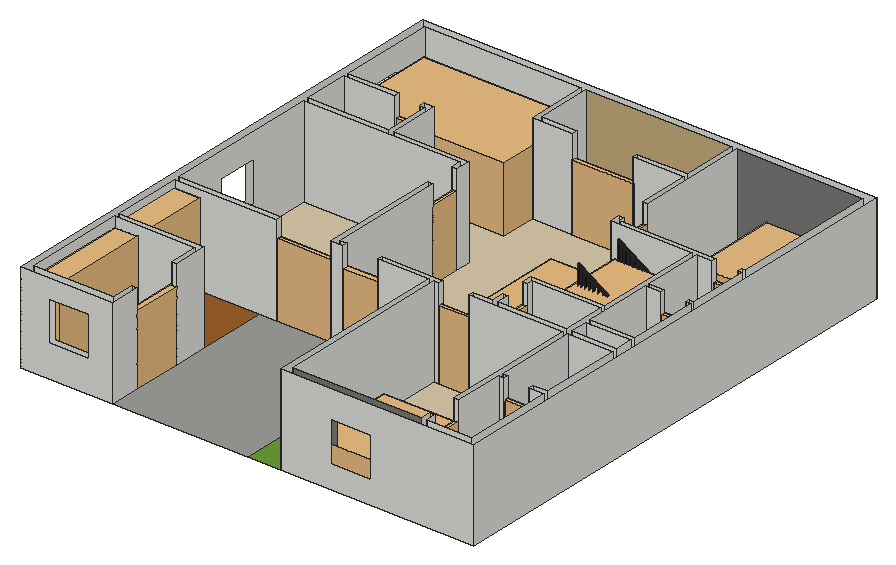
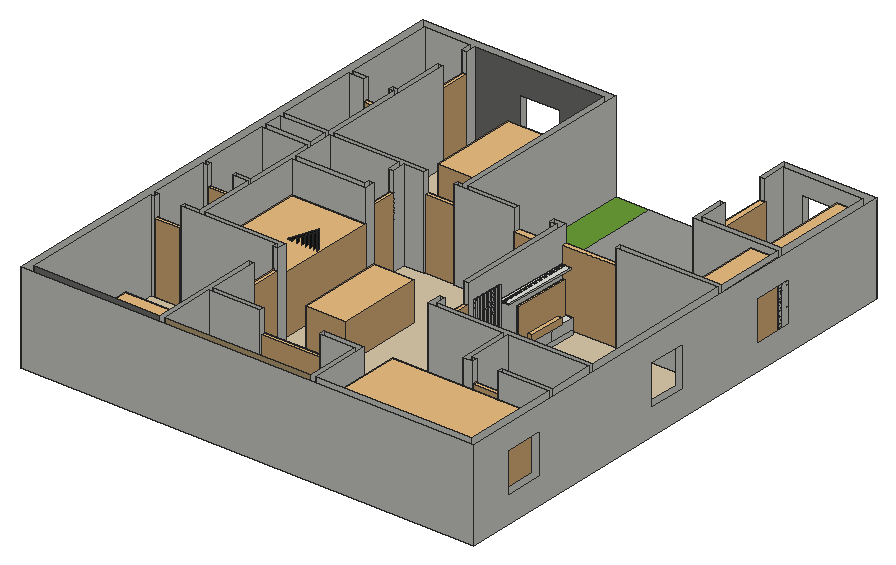
# SketchUp Ruby script. Lengths in inches.
U = 1.inch
M = Sketchup.active_model
def pt(a) = Geom::Point3d.new(a.map { |v| v * U })
def face(e, loops, mat)
  f = e.add_face(loops[0].map { |a| pt(a) })
  loops[1..].each { |l| e.add_face(l.map { |a| pt(a) }).erase! }
  f.material = f.back_material = mat if mat
  f
end
# faces: each face lists its corners as indices into pts; further lists are holes
def faces(e, pts, list, mat = nil) = list.each { |f| face(e, (f[0].is_a?(Array) ? f : [f]).map { |l| l.map { |i| pts[i] } }, mat) }
# xy, xz, yz: faces in a plane at the given z, y or x. An outline is a flat list of corners, or four numbers for a rectangle; further outlines are holes
def ring(l) = l.size == 4 ? [[l[0], l[1]], [l[2], l[1]], [l[2], l[3]], [l[0], l[3]]] : l.each_slice(2).to_a
def flat(e, list, mat, &to3) = list.each { |f| face(e, (f[0].is_a?(Array) ? f : [f]).map { |l| ring(l).map { |u, v| to3.(u, v) } }, mat) }
def xy(e, z, list, mat = nil) = flat(e, list, mat) { |x, y| [x, y, z] }
def xz(e, y, list, mat = nil) = flat(e, list, mat) { |x, z| [x, y, z] }
def yz(e, x, list, mat = nil) = flat(e, list, mat) { |y, z| [x, y, z] }
def lines(e, pts, list) = list.each { |a, b| e.add_line(pt(pts[a]), pt(pts[b])) }
# prism: a flat outline (further loops are holes) pulled along v
def prism(e, loops, v, mat = nil)
  f = face(e, loops, mat); d = Geom::Vector3d.new(v.map { |x| x * U })
  f.pushpull(f.normal.samedirection?(d) ? d.length : -d.length)
end
def box(e, o, s, mat = nil) = prism(e, [[o, [o[0] + s[0], o[1], o[2]], [o[0] + s[0], o[1] + s[1], o[2]], [o[0], o[1] + s[1], o[2]]]], [0, 0, s[2]], mat)
def at(x, y, z, deg = 0) = Geom::Transformation.translation(pt([x, y, z])) * Geom::Transformation.rotation(ORIGIN, Z_AXIS, deg.degrees)
def axes(o, x, y, z) = Geom::Transformation.new([*x, 0, *y, 0, *z, 0, *pt(o).to_a, 1])
def part(name) = M.definitions.add(name)
# library, detail: a bought-in or finely detailed component or shape, given as its bounding box
def library(name, o, s) = part(name).tap { |d| box(d.entities, o, s) }
def detail(e, o, s) = box(e.add_group.entities, o, s)
def put(e, d, t, mat = nil) = e.add_instance(d, t).tap { |i| i.material = mat if mat }
def group(e, t, mat = nil) = e.add_group.tap { |g| g.transformation = t; g.material = mat if mat }.entities
root = M.entities
M.materials.add("[Concrete Block 8x8 Gray]").color = [157, 158, 154]
M.materials.add("[Encaustic Tile Circular 01]").color = [123, 123, 122]
M.materials.add("[Field Square Tile]").color = [217, 201, 169]
M.materials.add("[Grass Dark Green]").color = [106, 157, 55]
M.materials.add("[Metal Panel]").color = [143, 157, 158]
M.materials.add("[Metal_Aluminum_Anodized]").color = [200, 209, 218]
M.materials.add("[Metal_Seamed]").color = [25, 25, 24]
M.materials.add("[Roofing Slate Tan]").color = [200, 175, 128]
M.materials.add("[Wood Floor Dark]").color = [153, 94, 42]
c1 = library("door",[0,0,0],[36,4.39,84])
c2 = library("double Door",[0,0,0],[79.98,10,87.99])
c3 = library("Gruppe\#1",[0,8.87,0],[102.36,152.23,141.73])
c4 = part("stairs, Holztreppe")
p = [[-31.58,140.69,125.98],[-31.58,140.71,125.98]]
lines(c4.entities,p,[[0,1]])
put(c4.entities,c3,axes([-51.18,-74.49,0],[1,0,0],[0,1,0],[0,0,0.77775]))
c5 = part("Group\#71")
box(c5.entities,[0,0,0],[1.97,1.22,32.37],"[Metal_Seamed]")
c6 = part("Group\#81")
box(c6.entities,[0,0,0],[1.97,51.19,3.0625],"[Metal_Seamed]")
c7 = part("Group\#76")
prism(c7.entities,[[[1.97,94.48,0],[1.97,94.48,3.0625],[1.97,0,58.18],[1.97,0,55.12]]],[-1.97,0,0],"[Metal_Seamed]")
c8 = part("Group\#74")
xz(c8.entities,0,[[0,0,1.97,33.27]],"[Metal_Seamed]")
xz(c8.entities,1.02,[[0,0,1.97,32.68]],"[Metal_Seamed]")
yz(c8.entities,0,[[0,0,0,33.27,1.02,32.68,1.02,0]],"[Metal_Seamed]")
yz(c8.entities,1.97,[[0,0,1.02,0,1.02,32.68,0,33.27]],"[Metal_Seamed]")
c9 = part("Group\#86")
box(c9.entities,[0,0,0],[1.18,1.97,32.37],"[Metal_Seamed]")
c10 = part("Untitled")
g1 = group(c10.entities,at(-2.72,-61.9,-3.0625))
g2 = group(g1,at(0,0,0))
put(g2,c4,at(53.15,65.62,3.0625))
g3 = group(g2,at(0,6.55,0))
g4 = group(g3,at(0,94.49,55.12))
xy(g4,0,[[104.33,0,106.3,51.19],[0,51.19,106.3,53.16]],"[Metal_Seamed]")
xy(g4,3.0625,[[104.33,0,106.3,8.07],[104.33,9.29,106.3,51.19],[0,51.19,106.3,53.16]],"[Metal_Seamed]")
xz(g4,0,[[104.33,0,106.3,3.0625]],"[Metal_Seamed]")
xz(g4,51.19,[[0,0,104.33,3.0625],[104.33,0,106.3,3.0625]],"[Metal_Seamed]")
xz(g4,53.16,[[0,0,106.3,3.0625]],"[Metal_Seamed]")
yz(g4,0,[[51.19,0,53.16,3.0625]],"[Metal_Seamed]")
yz(g4,104.33,[[0,0,51.19,3.0625]],"[Metal_Seamed]")
yz(g4,106.3,[[0,0,51.19,3.0625],[51.19,0,53.16,3.0625]],"[Metal_Seamed]")
put(g4,c5,at(104.33,8.07,3.0625))
put(g4,c5,at(104.33,19.6,3.0625))
put(g4,c5,at(104.33,30.24,3.0625))
put(g4,c5,at(104.33,40.72,3.0625))
put(g4,c5,at(104.33,51.95,3.0625))
put(g4,c5,at(0,51.89,3.0625))
put(g4,c5,at(0,8.01,3.0625))
put(g4,c5,at(0,19.54,3.0625))
put(g4,c5,at(0,40.66,3.0625))
put(g4,c5,at(0,30.18,3.0625))
put(g3,c6,at(0,94.49,55.12))
put(g3,c7,at(0,0.01,55.12))
g5 = group(g3,at(104.33,0.01,58.18))
prism(g5,[[[1.97,0,-55.12],[1.97,1.02,-54.52],[1.97,94.48,0],[1.97,94.48,-3.0625],[1.97,0,-58.18]]],[-1.97,0,0],"[Metal_Seamed]")
xy(g5,-21.84,[[0,0,1.97,1.02]],"[Metal_Seamed]")
put(g5,c8,axes([0,0,-21.84],[1,0,0],[0,1,0],[0,0,-1]))
put(g5,c8,axes([0,7.26,-17.61],[1,0,0],[0,1,0],[0,0,-1]))
put(g5,c8,axes([0,14.83,-13.19],[1,0,0],[0,1,0],[0,0,-1]))
put(g5,c8,axes([0,23.44,-8.17],[1,0,0],[0,1,0],[0,0,-1]))
put(g5,c8,axes([0,32.28,-3.01],[1,0,0],[0,1,0],[0,0,-1]))
put(g5,c8,axes([0,41.76,2.52],[1,0,0],[0,1,0],[0,0,-1]))
put(g5,c8,axes([0,51.4,8.14],[1,0,0],[0,1,0],[0,0,-1]))
put(g5,c8,axes([0,61.47,14.02],[1,0,0],[0,1,0],[0,0,-1]))
put(g5,c8,axes([0,72,20.16],[1,0,0],[0,1,0],[0,0,-1]))
put(g5,c8,axes([0,81.86,25.91],[1,0,0],[0,1,0],[0,0,-1]))
put(g5,c8,axes([0,93.45,32.68],[1,0,0],[0,1,0],[0,0,-1]))
put(g5,c8,axes([-49.33,51.4,8.14],[1,0,0],[0,1,0],[0,0,-1]))
put(g5,c8,axes([-49.33,93.45,32.68],[1,0,0],[0,1,0],[0,0,-1]))
put(g5,c8,axes([-49.33,0,-21.84],[1,0,0],[0,1,0],[0,0,-1]))
put(g5,c8,axes([-49.33,41.76,2.52],[1,0,0],[0,1,0],[0,0,-1]))
put(g5,c8,axes([-49.33,72,20.16],[1,0,0],[0,1,0],[0,0,-1]))
put(g5,c8,axes([-49.33,32.28,-3.01],[1,0,0],[0,1,0],[0,0,-1]))
put(g5,c8,axes([-49.33,23.44,-8.17],[1,0,0],[0,1,0],[0,0,-1]))
put(g5,c8,axes([-49.33,81.86,25.91],[1,0,0],[0,1,0],[0,0,-1]))
put(g5,c8,axes([-49.33,14.83,-13.19],[1,0,0],[0,1,0],[0,0,-1]))
put(g5,c8,axes([-49.33,61.47,14.02],[1,0,0],[0,1,0],[0,0,-1]))
put(g5,c8,axes([-49.33,7.26,-17.61],[1,0,0],[0,1,0],[0,0,-1]))
put(g5,c8,at(-104.33,93.45,-0.18))
put(g5,c8,at(-104.33,23.44,40.66))
put(g5,c8,at(-104.33,7.26,50.11))
put(g5,c8,at(-104.33,72,12.34))
put(g5,c8,at(-104.33,32.28,35.51))
put(g5,c8,at(-104.33,0,54.34))
put(g5,c8,at(-104.33,81.86,6.59))
put(g5,c8,at(-104.33,14.83,45.6875))
put(g5,c8,at(-104.33,61.47,18.48))
put(g5,c8,at(-104.33,41.76,29.97))
put(g5,c8,at(-104.33,51.4,24.35))
put(g5,c8,at(-55.12,23.43,40.26))
put(g5,c8,at(-55.12,81.84,6.18))
put(g5,c8,at(-55.12,7.24,49.7))
put(g5,c8,at(-55.12,-0.01,53.93))
put(g5,c8,at(-55.12,41.75,29.57))
put(g5,c8,at(-55.12,61.46,18.07))
put(g5,c8,at(-55.12,93.44,-0.59))
put(g5,c8,at(-55.12,32.27,35.1))
put(g5,c8,at(-55.12,51.39,23.95))
put(g5,c8,at(-55.12,14.8125,45.29))
put(g5,c8,at(-55.12,71.98,11.93))
put(g3,c7,at(49.21,0,55.12))
put(g3,c7,axes([55,0.01,58.18],[1,0,0],[0,1,0],[0,0,-1]))
g6 = group(g2,at(0,6.55,35.43))
p = [[51.18,94.48,55.12],[51.18,94.48,58.18],[55,94.49,58.18],[55,94.49,55.12]]
faces(g6,p,[[0,1,2,3]],"[Metal_Seamed]")
g7 = group(g6,at(0,94.49,55.12))
xy(g7,0,[[104.33,0,106.3,51.19],[0,51.19,106.3,53.16]],"[Metal_Seamed]")
xy(g7,3.0625,[[104.33,0,106.3,51.19],[0,51.19,106.3,53.16]],"[Metal_Seamed]")
xz(g7,0,[[104.33,0,106.3,3.0625]],"[Metal_Seamed]")
xz(g7,51.19,[[0,0,104.33,3.0625],[104.33,0,106.3,3.0625]],"[Metal_Seamed]")
xz(g7,53.16,[[0,0,106.3,3.0625]],"[Metal_Seamed]")
yz(g7,0,[[51.19,0,53.16,3.0625]],"[Metal_Seamed]")
yz(g7,104.33,[[0,0,51.19,3.0625]],"[Metal_Seamed]")
yz(g7,106.3,[[0,0,51.19,3.0625],[51.19,0,53.16,3.0625]],"[Metal_Seamed]")
put(g6,c6,at(0,94.49,55.12))
put(g6,c7,at(0,0.01,55.12))
put(g6,c7,axes([104.33,0.01,58.18],[1,0,0],[0,1,0],[0,0,-1]))
put(g6,c7,at(49.21,0,55.12))
put(g6,c7,axes([55,0.01,58.18],[1,0,0],[0,1,0],[0,0,-1]))
put(g1,c9,at(94.51,152.23,58.18))
put(g1,c9,at(48.39,152.23,58.18))
put(g1,c9,at(21.29,152.23,58.18))
put(g1,c9,at(85.01,152.23,58.18))
put(g1,c9,at(58.09,152.23,58.18))
put(g1,c9,at(75.58,152.23,58.18))
put(g1,c9,at(66.57,152.23,58.18))
put(g1,c9,at(38.93,152.23,58.18))
put(g1,c9,at(10.71,152.23,58.18))
put(g1,c9,at(29.75,152.23,58.18))
c11 = library("sliding+window",[0,-1.1,0],[78.74,4.33,80.71])
c12 = library("door1",[3.7,-4.82,1.36],[53.55,7.65,83.26])
c13 = library("bed",[-16.91,-10.3,-0.31],[85.22,91.2,40.45])
c14 = library("04 tu bep",[0,0,0],[96.93,181.8125,106.3])
c15 = library("Sitting+set",[-42.84,56.36,0],[31.38,80.81,100.21])
c16 = library("Pujaa 1",[0,0,0],[26.5,60,96])
c17 = library("sofa",[-1.18,-2.36,0],[94.72,146.45,38.04])
c18 = part("Agrupar\#1")
detail(c18.entities,[0,0,0],[43.31,13.99,7.25])
c19 = library("Agrupar\#2",[0,0,0],[66.49,2.6,38.28])
c20 = part("Samsung 75")
p = [[0,0,0],[1,0,0],[1,1,0]]
lines(c20.entities,p,[[0,1],[1,2],[2,0]])
put(c20.entities,c18,at(200.625,110.82,-2.44),"[Metal_Aluminum_Anodized]")
put(c20.entities,c19,at(189.03,116.54,0))
c21 = library("Vtufgjkbc",[-37.34,-38.3,0],[76.68,71.13,141.17])
c22 = part("Enscape.LinearLight")
xz(c22.entities,-44.64,[[0,-1,0,0,-0.38,-0.92],[0,-1,0.38,-0.92,0,0],[-0.38,-0.92,0,0,-0.71,-0.71],[0.38,-0.92,0.71,-0.71,0,0],[-0.71,-0.71,0,0,-0.92,-0.38],
  [0.71,-0.71,0.92,-0.38,0,0],[-0.92,-0.38,0,0,-1,0],[0.92,-0.38,1,0,0,0],[-1,0,0,0,-0.92,0.38],[0,0,-0.71,0.71,-0.92,0.38],
  [0,0,-0.38,0.92,-0.71,0.71],[0,0,0,1,-0.38,0.92],[0,0,0.38,0.92,0,1],[0,0,0.71,0.71,0.38,0.92],[0,0,0.92,0.38,0.71,0.71],
  [0,0,1,0,0.92,0.38]])
xz(c22.entities,44.64,[[0,-1,-0.38,-0.92,0,0],[0,-1,0,0,0.38,-0.92],[-0.38,-0.92,-0.71,-0.71,0,0],[0.38,-0.92,0,0,0.71,-0.71],[-0.71,-0.71,-0.92,-0.38,0,0],
  [0.71,-0.71,0,0,0.92,-0.38],[-0.92,-0.38,-1,0,0,0],[0.92,-0.38,0,0,1,0],[-1,0,-0.92,0.38,0,0],[0,0,-0.92,0.38,-0.71,0.71],
  [0,0,-0.71,0.71,-0.38,0.92],[0,0,-0.38,0.92,0,1],[0,0,0,1,0.38,0.92],[0,0,0.38,0.92,0.71,0.71],[0,0,0.71,0.71,0.92,0.38],
  [0,0,0.92,0.38,1,0]])
p = [[-0.38,-44.64,-0.92],[-0.38,44.64,-0.92],[0,44.64,-1],[0,-44.64,-1],[0.38,44.64,-0.92],[0.38,-44.64,-0.92],
  [-0.71,-44.64,-0.71],[-0.71,44.64,-0.71],[0.71,44.64,-0.71],[0.71,-44.64,-0.71],[-0.92,-44.64,-0.38],[-0.92,44.64,-0.38],
  [0.92,44.64,-0.38],[0.92,-44.64,-0.38],[-1,-44.64,0],[-1,44.64,0],[1,44.64,0],[1,-44.64,0],
  [-0.92,-44.64,0.38],[-0.92,44.64,0.38],[0.92,44.64,0.38],[0.92,-44.64,0.38],[-0.71,-44.64,0.71],[-0.71,44.64,0.71],
  [0.71,44.64,0.71],[0.71,-44.64,0.71],[-0.38,-44.64,0.92],[-0.38,44.64,0.92],[0.38,44.64,0.92],[0.38,-44.64,0.92],
  [0,-44.64,1],[0,44.64,1]]
faces(c22.entities,p,[[0,1,2],[0,2,3],[3,2,4],[3,4,5],[6,7,1],[6,1,0],[5,4,8],[5,8,9],
  [10,11,7],[10,7,6],[9,8,12],[9,12,13],[14,15,11],[14,11,10],[13,12,16],[13,16,17],
  [18,19,15],[18,15,14],[17,16,20],[17,20,21],[22,23,19],[22,19,18],[21,20,24],[21,24,25],
  [26,27,23],[26,23,22],[25,24,28],[25,28,29],[30,31,27],[30,27,26],[29,28,31],[29,31,30]])
c23 = part("Group\#8")
box(c23.entities,[0,0,0],[1.57,1.18,81.22])
c24 = part("tv unit")
put(c24.entities,c20,at(-134.98,-45.95,38.54))
put(c24.entities,c21,axes([23.51,76.07,18.38],[0.185,0,0],[0,0.185,0],[0,0,0.185]))
put(c24.entities,c22,axes([87.75,81.2,82.67],[-0.0192,0.99911,-0.03748],[-0.99982,-0.01919,0.00072],[0,0.03749,0.9993]))
g8 = group(c24.entities,at(3.9375,84.65,12.68))
box(g8,[0,-13.78,0],[127.95,13.78,5.79])
g9 = group(c24.entities,at(43.31,84.65,18.46))
prism(g9,[[[0,0,0],[88.58,0,0],[88.58,-13.78,0],[59.21,-13.78,0],[59.21,-12.99,0],[59.06,-12.99,0],[59.06,-13.78,0],[29.69,-13.78,0],[29.69,-12.99,0],[29.53,-12.99,0],[29.53,-13.78,0],[0,-13.78,0]]],[0,0,12.6])
g10 = group(c24.entities,at(3.9375,84.65,18.46))
put(g10,c23,at(0,-1.18,0))
g11 = group(g10,at(1.97,-1.18,0))
box(g11,[0,0,0],[1.57,1.18,81.22])
put(g10,c23,at(3.9375,-1.18,0))
put(g10,c23,at(5.91,-1.18,0))
g12 = group(g10,at(7.875,-1.18,0))
box(g12,[0,0,0],[1.57,1.18,81.22])
put(g10,c23,at(9.84,-1.18,0))
put(g10,c23,at(11.8125,-1.18,0))
put(g10,c23,at(13.78,-1.18,0))
put(g10,c23,at(15.75,-1.18,0))
put(g10,c23,at(17.72,-1.18,0))
put(g10,c23,at(19.69,-1.18,0))
put(g10,c23,at(21.65,-1.18,0))
put(g10,c23,at(23.62,-1.18,0))
g13 = group(g10,at(25.59,-1.18,0))
box(g13,[0,0,0],[1.57,1.18,81.22])
put(g10,c23,at(27.56,-1.18,0))
put(g10,c23,at(29.53,-1.18,0))
put(g10,c23,at(31.5,-1.18,0))
put(g10,c23,at(33.46,-1.18,0))
put(g10,c23,at(35.43,-1.18,0))
put(g10,c23,at(37.4,-1.18,0))
g14 = group(c24.entities,at(42.91,84.65,81.97))
box(g14,[0,-11.8125,0],[88.98,11.8125,1.97])
xy(root,0,[[[0,0,110,0,110,36.625,104,36.625,104,9,9,9,9,130,104,130,104,95.625,110,95.625,110,136,9,136,9,219,130,219,130,225,9,225,9,411,195,411,195,399,201,399,201,417,111,417,111,477,99,477,99,471,105,471,105,417,9,417,9,471,69,471,69,477,9,477,9,591,195,591,195,519,243.14,519,243.14,525,201,525,201,591,375,591,375,525,315.14,525,315.14,519,375,519,375,459,381,459,381,591,531,591,531,417,526.66,417,526.66,411,531,411,531,340,525,340,525,335,531,335,531,252,477,252,477,335,495,335,495,340,477,340,477,411,495.74,411,495.74,417,381,417,381,423,375,423,375,411,471,411,471,282,383,282,383,270,389,270,389,276,471,276,471,225,389,225,389,240,383,240,383,225,359,225,359,219,471,219,471,57,477,57,477,116,483,116,483,122,477,122,477,219,531,219,531,122,513,122,513,116,531,116,531,9,477,9,477,21,471,21,471,9,317,9,317,219,323,219,323,225,250.53,225,250.53,219,311,219,311,0,540,0,540,600,0,600],[477,225,531,246]],[195,219,195,363,201,363,201,225,208.87,225,208.87,219],[477,225,531,246]])
xy(root,0,[[110,0,271.37,219]],"[Concrete Block 8x8 Gray]")
xy(root,0,[[317,9,471,9,471,21,477,21,477,9,531,9,531,116,477,116,477,57,471,57,471,219,359,219,359,225,383,225,383,282,471,282,471,411,375,411,375,423,381,423,381,417,531,417,531,591,381,591,381,459,375,459,375,519,195,519,195,591,9,591,9,477,111,477,111,417,201,417,201,399,195,399,195,411,9,411,9,225,130,225,130,219,195,219,195,363,201,363,201,225,208.87,225,208.87,219,250.53,219,250.53,225,323,225,323,219,317,219],[9,9,104,9,104,36.625,110,36.625,110,95.625,104,95.625,104,130,9,130]],"[Field Square Tile]")
xy(root,0,[[271.37,0,311,219],[243.14,519,315.14,519,315.14,525,375,525,375,591,201,591,201,525,243.14,525]],"[Grass Dark Green]")
xy(root,0,[[483,116,513,116,513,122,531,122,531,219,477,219,477,122,483,122],[389,225,471,225,471,276,389,276,389,270,383,270,383,240,389,240],[477,252,531,252,531,335,525,335,525,340,531,340,531,411,526.66,411,526.66,417,495.74,417,495.74,411,477,411,477,340,495,340,495,335,477,335],[9,417,105,417,105,471,99,471,99,477,69,477,69,471,9,471]],"[Metal Panel]")
xy(root,0,[[9,136,110,219]],"[Wood Floor Dark]")
xz(root,0,[[[0,0,110,108],[33.63,38.11,81.63,86.11]],[[311,0,540,108],[370.05,27.37,418.05,75.37]]])
xz(root,9,[[[9,0,104,108],[33.63,38.11,81.63,86.11]],[477,0,531,108]])
xz(root,9,[[[317,0,471,108],[370.05,27.37,418.05,75.37]]],"[Encaustic Tile Circular 01]")
xz(root,21,[[471,0,477,108]])
xz(root,36.625,[[104,0,110,108]])
xz(root,57,[[471,0,477,108]])
xz(root,95.625,[[104,0,110,108]])
xz(root,116,[[477,0,483,108],[513,0,531,108]])
xz(root,122,[[477,0,483,108],[513,0,531,108]])
xz(root,130,[[9,0,104,108]])
xz(root,136,[[9,0,110,108]])
xz(root,219,[[9,0,130,108],[195,0,208.87,108],[250.53,0,311,108],[317,0,323,108],[359,0,471,108],
  [477,0,531,108]])
xz(root,225,[[9,0,130,108],[201,0,208.87,108],[250.53,0,323,108],[359,0,383,108],[389,0,471,108],
  [477,0,531,108]])
xz(root,240,[[383,0,389,108]])
xz(root,246,[[477,0,531,108]])
xz(root,252,[[477,0,531,108]])
xz(root,270,[[383,0,389,108]])
xz(root,276,[[389,0,471,108]])
xz(root,282,[[383,0,471,108]])
xz(root,335,[[477,0,495,108],[525,0,531,108]])
xz(root,340,[[477,0,495,108],[525,0,531,108]])
xz(root,363,[[195,0,201,108]])
xz(root,399,[[195,0,201,108]])
xz(root,411,[[9,0,195,108],[375,0,471,108],[477,0,495.74,108],[526.66,0,531,108]])
xz(root,417,[[9,0,105,108],[111,0,201,108],[381,0,495.74,108],[526.66,0,531,108]])
xz(root,423,[[375,0,381,108]])
xz(root,459,[[375,0,381,108]])
xz(root,471,[[9,0,69,108],[99,0,105,108]])
xz(root,477,[[9,0,69,108],[99,0,111,108]])
xz(root,519,[[195,0,243.14,108],[315.14,0,375,108]])
xz(root,525,[[201,0,243.14,108],[315.14,0,375,108]])
xz(root,591,[[9,0,195,108]])
xz(root,591,[[381,0,531,108]],"[Encaustic Tile Circular 01]")
xz(root,591,[[201,0,375,108]],"[Roofing Slate Tan]")
xz(root,600,[[0,0,540,108]])
yz(root,0,[[[0,0,600,108],[501.46,30.79,549.46,78.79],[288.02,30.79,336.02,78.79],[130.58,30.79,178.58,78.79]]])
yz(root,9,[[9,0,130,108],[136,0,219,0,219,108,136,108,136,78.79,178.58,78.79,178.58,30.79,136,30.79],[[225,0,411,108],[288.02,30.79,336.02,78.79]],[417,0,471,108],[[477,0,591,108],[501.46,30.79,549.46,78.79]]])
yz(root,69,[[471,0,477,108]])
yz(root,99,[[471,0,477,108]])
yz(root,104,[[9,0,36.625,108],[95.625,0,130,108]])
yz(root,105,[[417,0,471,108]])
yz(root,110,[[0,0,36.625,108],[95.625,0,136,108]])
yz(root,111,[[417,0,477,108]])
yz(root,130,[[219,0,225,108]])
yz(root,195,[[219,0,363,108],[399,0,411,108],[519,0,591,108]])
yz(root,201,[[225,0,363,108],[399,0,417,108],[525,0,591,108]])
yz(root,208.87,[[219,0,225,108]])
yz(root,243.14,[[519,0,525,108]])
yz(root,250.53,[[219,0,225,108]])
yz(root,311,[[0,0,219,108]])
yz(root,315.14,[[519,0,525,108]])
yz(root,317,[[9,0,219,108]])
yz(root,323,[[219,0,225,108]])
yz(root,359,[[219,0,225,108]])
yz(root,375,[[411,0,423,108],[459,0,519,108],[525,0,591,108]])
yz(root,381,[[417,0,423,108],[459,0,591,108]])
yz(root,383,[[225,0,240,108],[270,0,282,108]])
yz(root,389,[[225,0,240,108],[270,0,276,108]])
yz(root,471,[[9,0,21,108],[57,0,219,108],[225,0,276,108],[282,0,411,108]])
yz(root,477,[[9,0,21,108],[57,0,116,108],[122,0,219,108],[225,0,246,108],[252,0,335,108],
  [340,0,411,108]])
yz(root,483,[[116,0,122,108]])
yz(root,495,[[335,0,340,108]])
yz(root,495.74,[[411,0,417,108]])
yz(root,513,[[116,0,122,108]])
yz(root,525,[[335,0,340,108]])
yz(root,526.66,[[411,0,417,108]])
yz(root,531,[[9,0,116,108],[122,0,219,108],[225,0,246,108],[252,0,335,108],[340,0,411,108],
  [417,0,591,108]])
yz(root,540,[[0,0,600,108]])
put(root,c1,axes([483,117.61,0],[0.83333,0,0],[0,1,0],[0,0,1]))
put(root,c1,axes([69,472.61,0],[0.83333,0,0],[0,1,0],[0,0,1]))
put(root,c1,at(201,363,0,90))
put(root,c2,axes([130,219,0],[0.81274,0,0],[0,0.5,0],[0,0,1]))
put(root,c1,at(475.39,21,0,90))
put(root,c1,at(379.39,423,0,90))
put(root,c1,axes([383,270,0],[0,-0.83333,0],[1,0,0],[0,0,1]))
put(root,c10,axes([416.82,407.71,1.91],[0,-1.21356,0],[0.5777,0,0],[0,0,0.6248]))
put(root,c11,axes([243.14,519,0],[0.9303,0,0],[0,1,0],[0,0,1]))
put(root,c12,axes([205.99,223.82,-1.36],[0.77801,0,0],[0,1,0],[0,0,1]))
put(root,c12,axes([105.18,32.55,-1.36],[0,1.1018,0],[-1,0,0],[0,0,1]))
put(root,c1,axes([496.66,412.61,0],[0.83333,0,0],[0,1,0],[0,0,1]))
put(root,c13,axes([413.57,102.4375,0.33],[-1.05,0,0],[0,-1.155,0],[0,0,1.05]))
put(root,c14,axes([10.55,587.47,0],[0,-1.13966,0],[1.01449,0,0],[0,0,0.7316]))
put(root,c15,at(51.74,80.1,0))
put(root,c16,axes([35.5,130,0],[-1,0,0],[0,-1.93591,0],[0,0,1]))
put(root,c1,axes([495,335.61,0],[0.83333,0,0],[0,1,0],[0,0,1]))
put(root,c1,at(323,219,0))
put(root,c13,axes([434.62,497.5625,0.33],[1.05,0,0],[0,1.155,0],[0,0,1.05]))
put(root,c17,axes([354.27,404.83,0],[-0.50388,0,0],[0,-0.697,0],[0,0,1.2155]))
put(root,c24,at(110.5,364.01,-12.68,-91.6))
